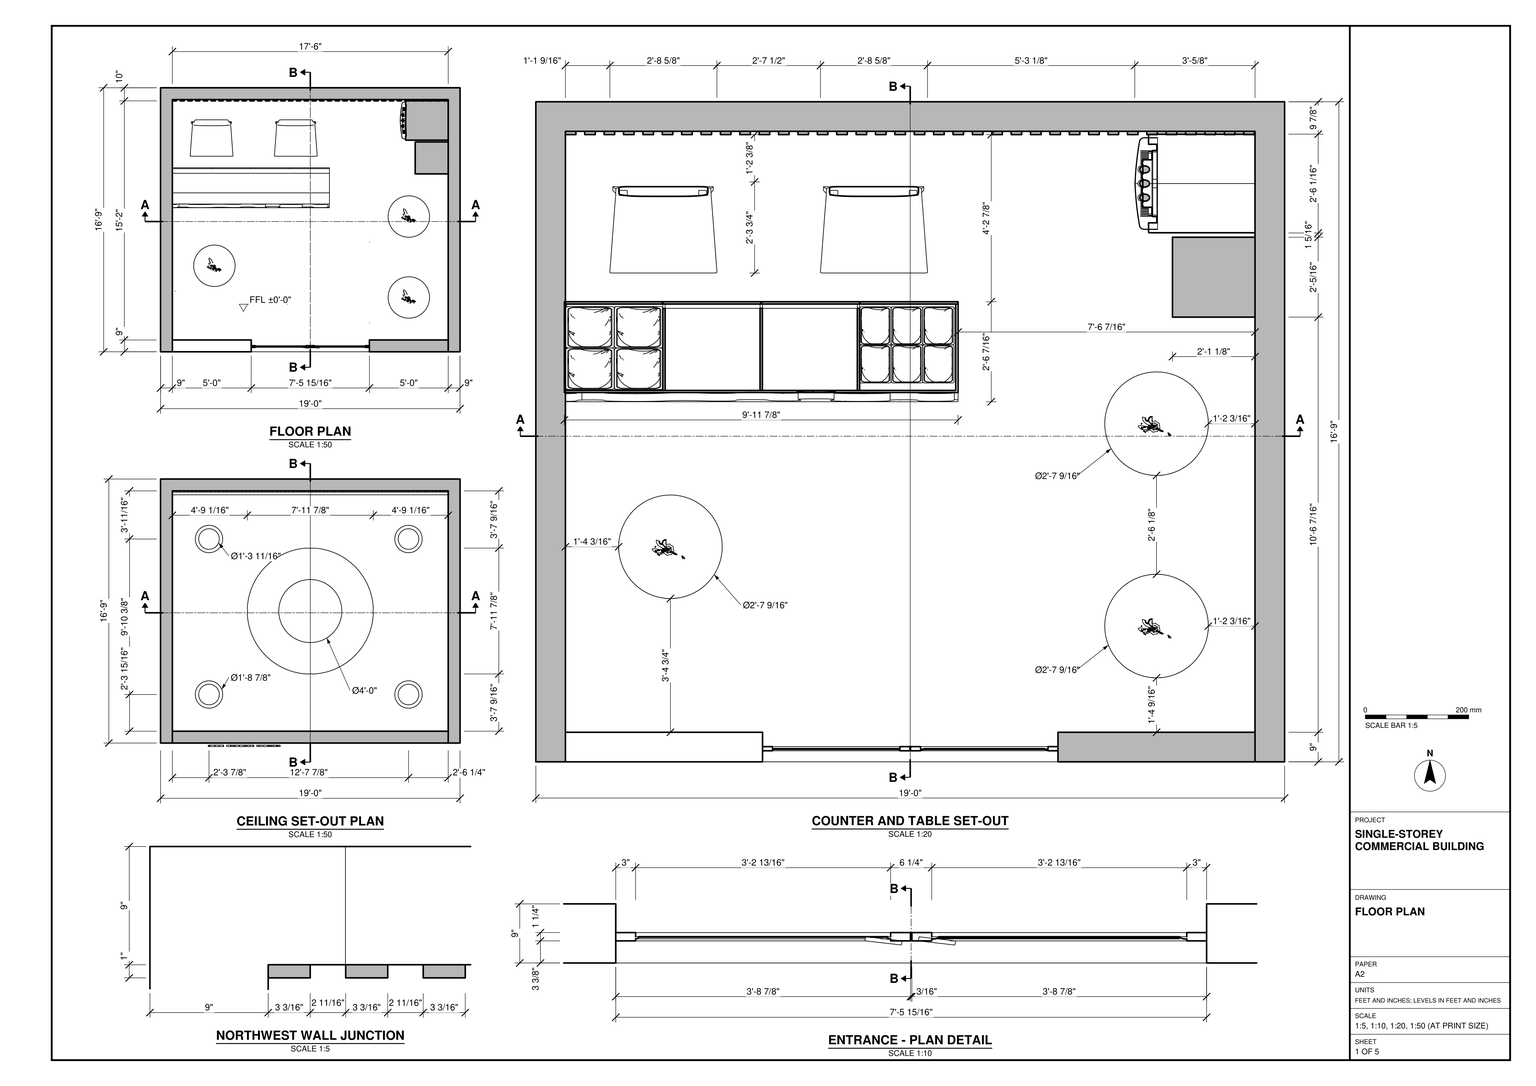
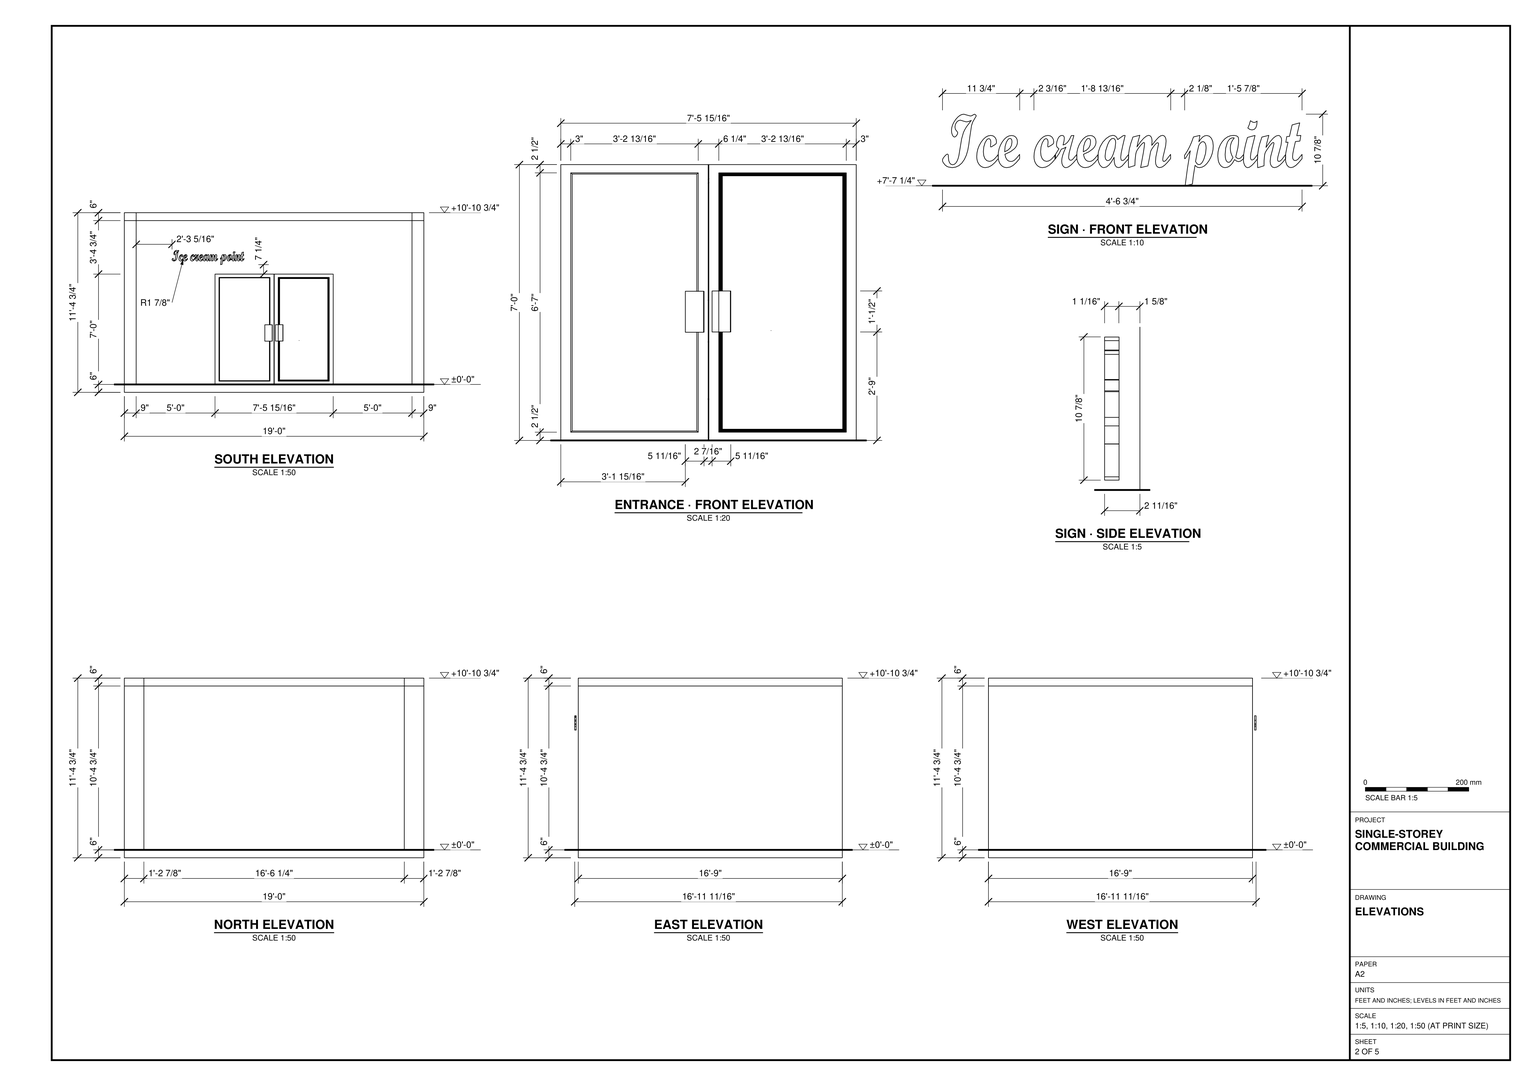
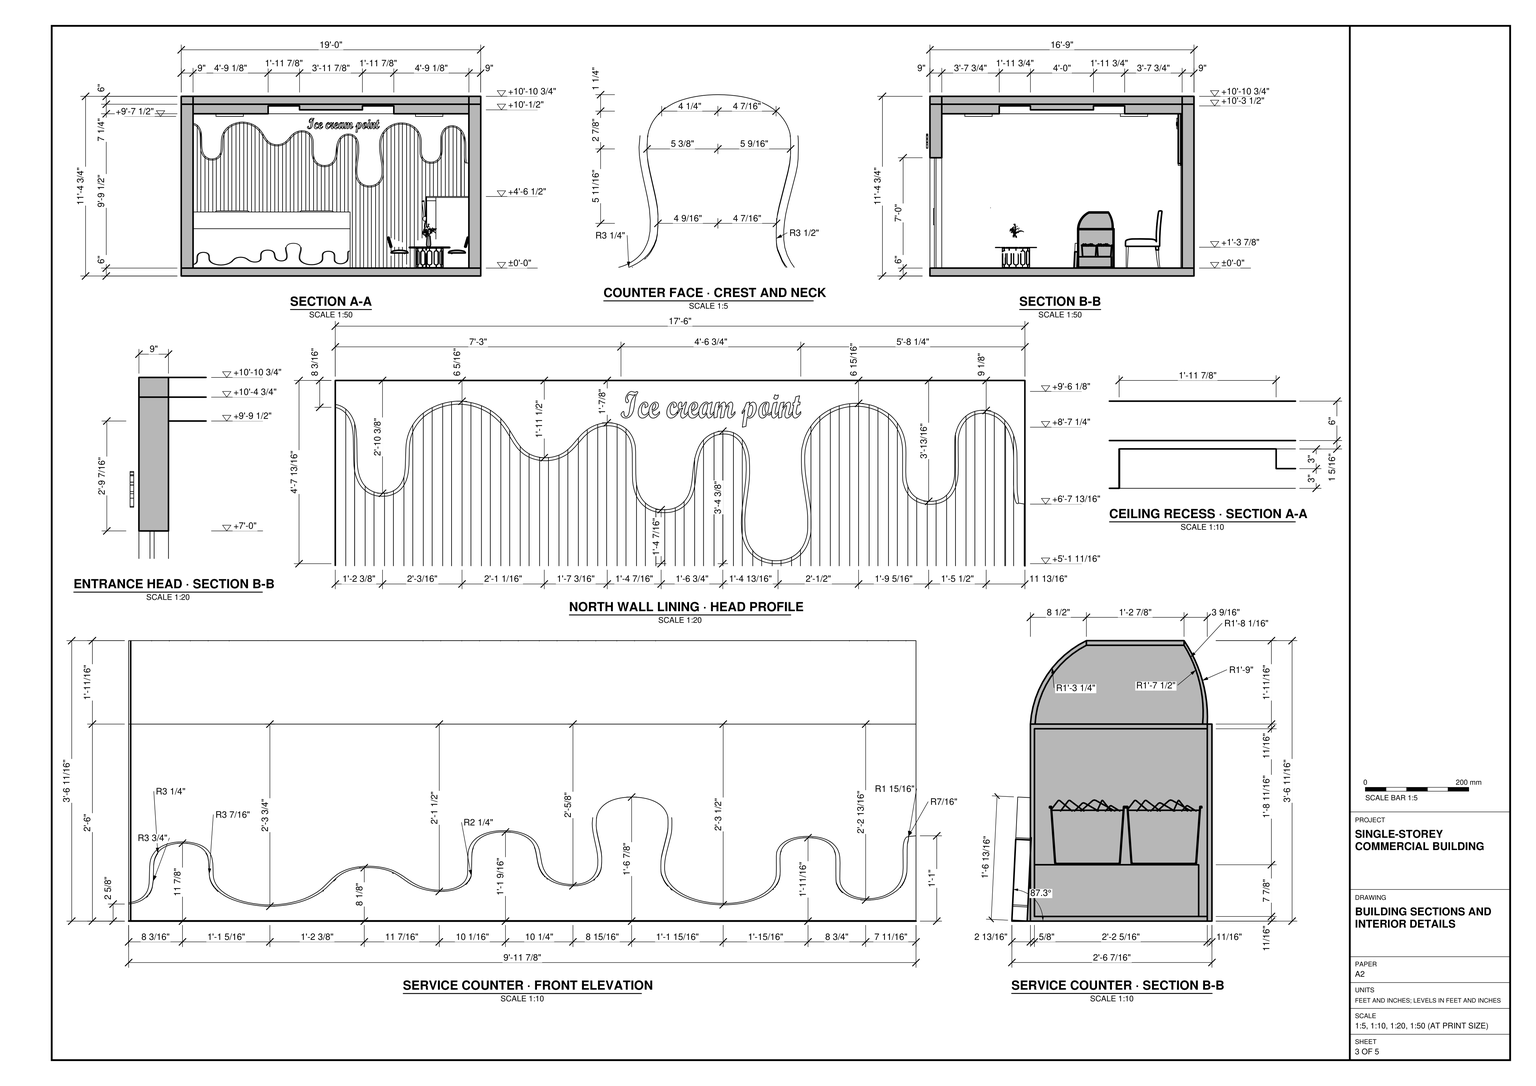
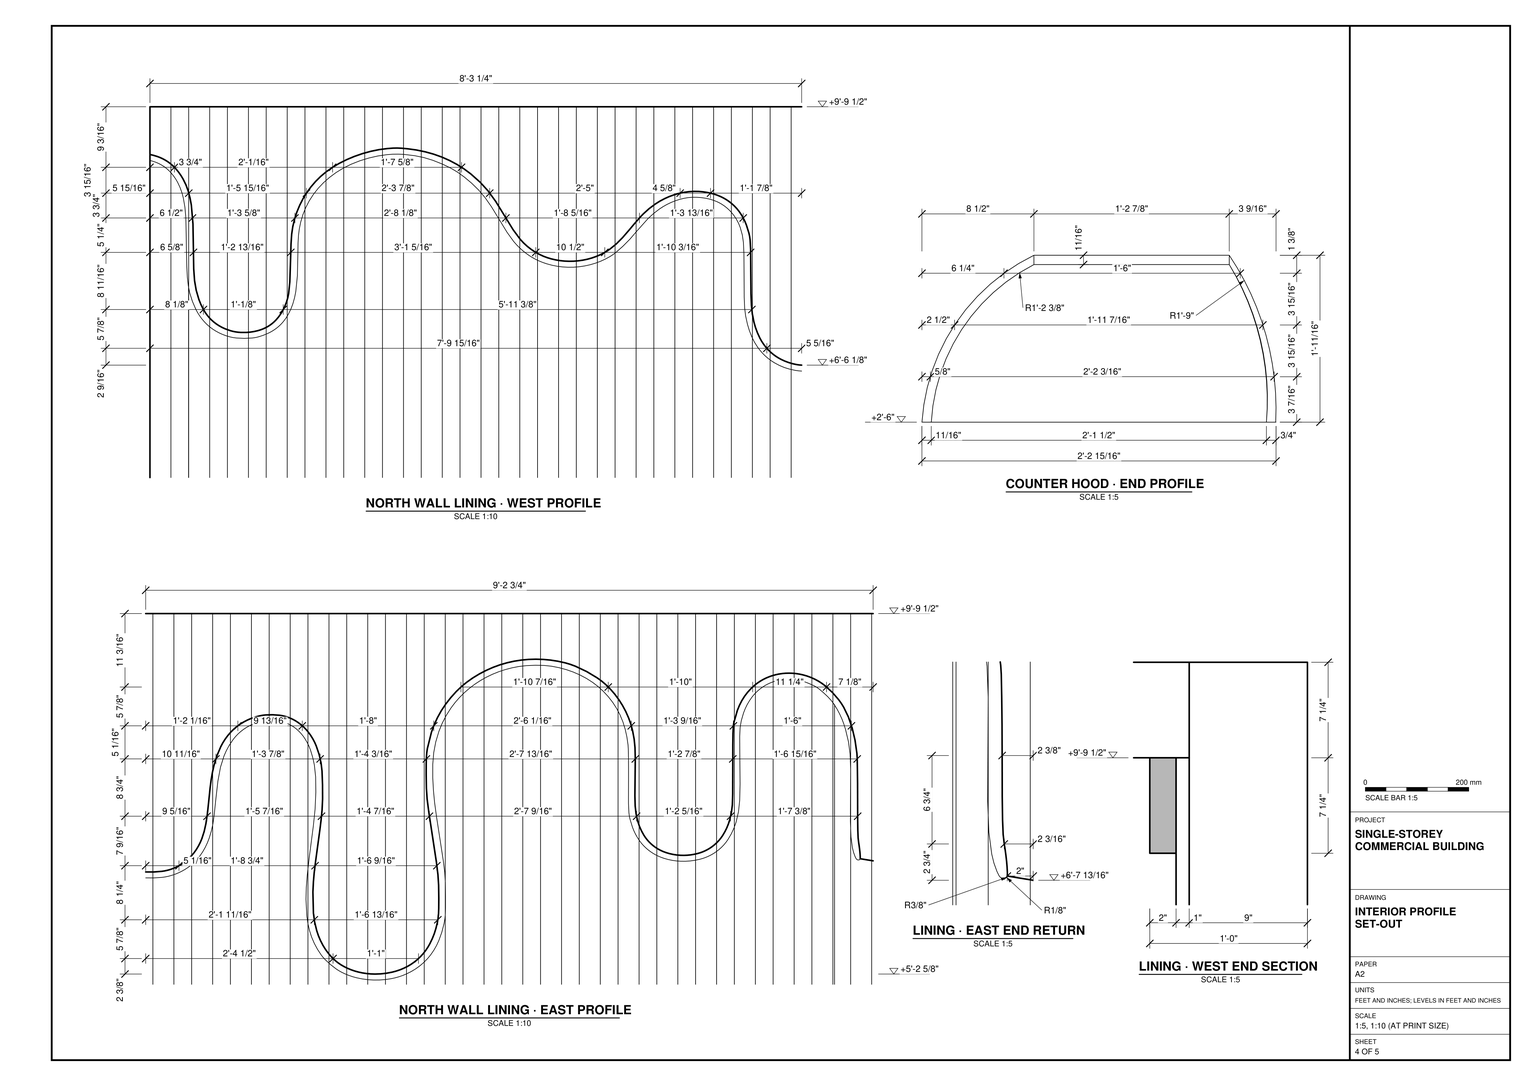
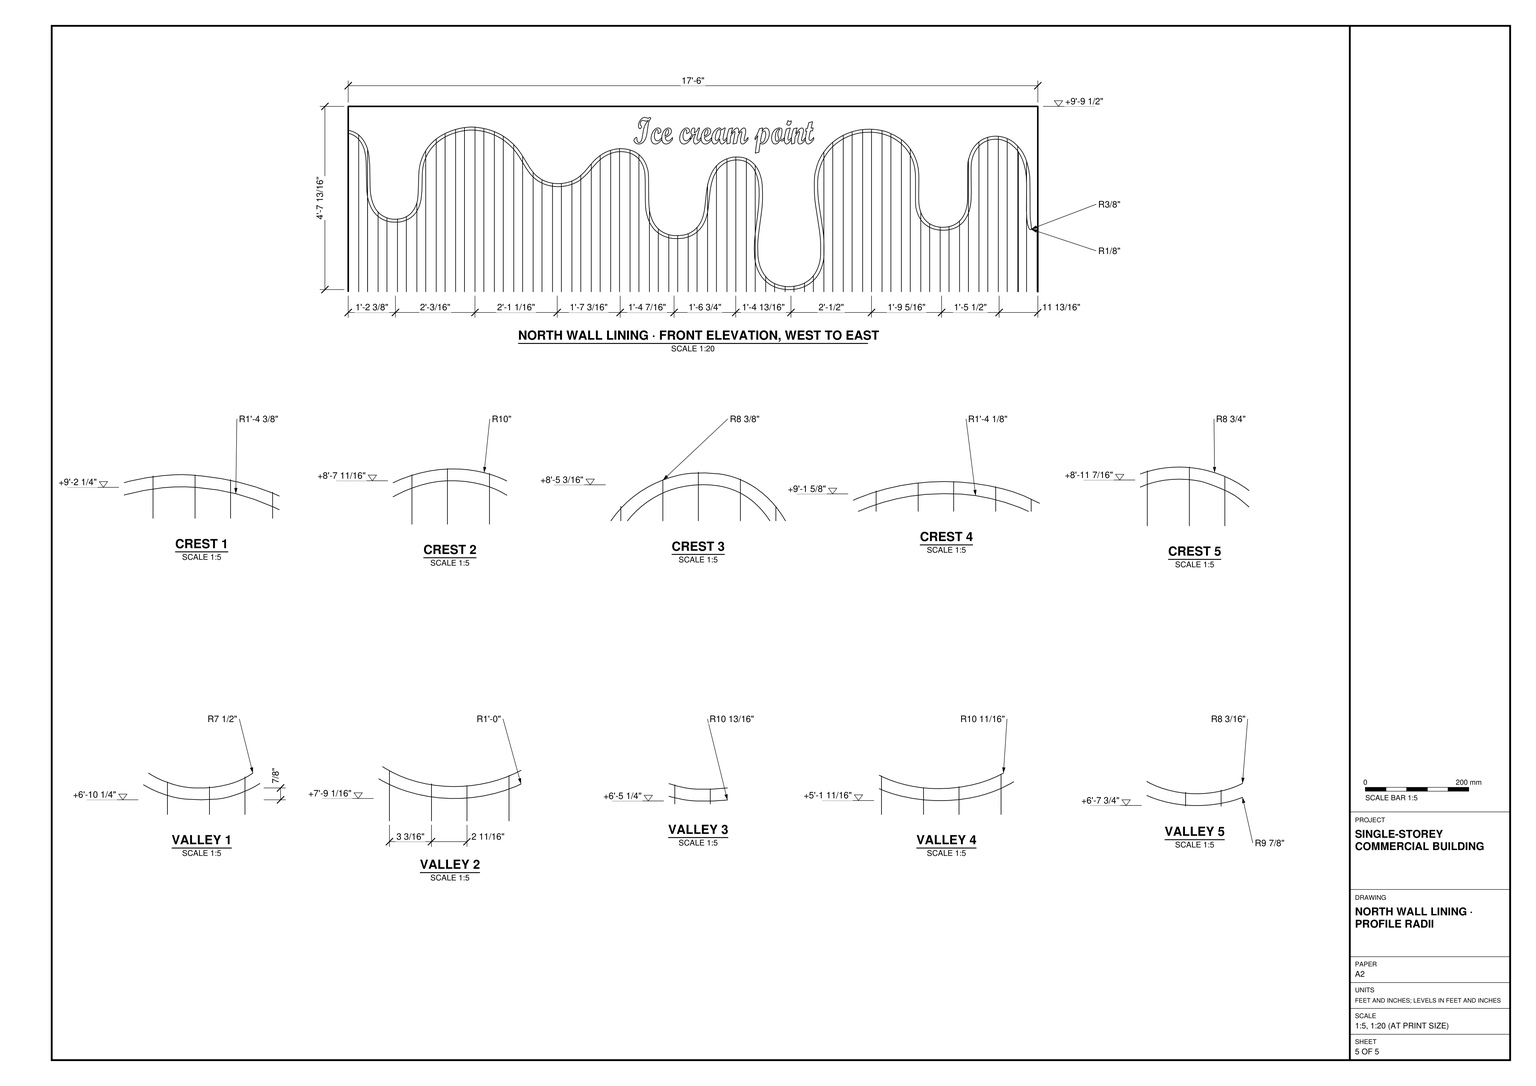
Build the ice cream shop in SketchUp from task_files/diagram_01.pdf. Work in feet and inches. The finished model, including the projecting entrance sign, must measure 19'-0" east to west, 16'-11 11/16" north to south and 11'-4 3/4" high. Set the single finished floor level at ±0'-0".

Build the floor slab, perimeter walls and flat roof slab. Use the wall thicknesses and north wall lining detail shown in plan. Centre the pair of framed entrance doors in the south wall, with pulls at the meeting edges. Place the exterior lettering above and to the left of the centre of the entrance as shown in elevation.

Use the counter and table set-out to arrange the interior. Run the display counter eastward from the west wall, leaving space for the two chairs between the counter and the north wall. Model the rounded display cover, the tubs and the undulating profile on the counter face. Behind it, form the full-width vertical wall lining with its varying curved head and interior lettering. Include the equipment and adjacent unit at the northeast corner. Place the three round tables in the customer area and reproduce the central and four surrounding circular features in the ceiling set-out.

Keep shell elements and each piece of furniture or joinery in separate groups or components, and use components for repeated parts. Decor and loose items may be any suitable library components. Save one SketchUp model as output_files/single_storey_ice_cream_shop_and_its_service_counter.skp.

# SketchUp Ruby script. Lengths in inches.
U = 1.inch
M = Sketchup.active_model
def pt(a) = Geom::Point3d.new(a.map { |v| v * U })
def face(e, loops, mat)
  f = e.add_face(loops[0].map { |a| pt(a) })
  loops[1..].each { |l| e.add_face(l.map { |a| pt(a) }).erase! }
  f.material = f.back_material = mat if mat
  f
end
# faces: each face lists its corners as indices into pts; further lists are holes
def faces(e, pts, list, mat = nil) = list.each { |f| face(e, (f[0].is_a?(Array) ? f : [f]).map { |l| l.map { |i| pts[i] } }, mat) }
# xy, xz, yz: faces in a plane at the given z, y or x. An outline is a flat list of corners, or four numbers for a rectangle; further outlines are holes
def ring(l) = l.size == 4 ? [[l[0], l[1]], [l[2], l[1]], [l[2], l[3]], [l[0], l[3]]] : l.each_slice(2).to_a
def flat(e, list, mat, &to3) = list.each { |f| face(e, (f[0].is_a?(Array) ? f : [f]).map { |l| ring(l).map { |u, v| to3.(u, v) } }, mat) }
def xy(e, z, list, mat = nil) = flat(e, list, mat) { |x, y| [x, y, z] }
def xz(e, y, list, mat = nil) = flat(e, list, mat) { |x, z| [x, y, z] }
def yz(e, x, list, mat = nil) = flat(e, list, mat) { |y, z| [x, y, z] }
def lines(e, pts, list) = list.each { |a, b| e.add_line(pt(pts[a]), pt(pts[b])) }
# prism: a flat outline (further loops are holes) pulled along v
def prism(e, loops, v, mat = nil)
  f = face(e, loops, mat); d = Geom::Vector3d.new(v.map { |x| x * U })
  f.pushpull(f.normal.samedirection?(d) ? d.length : -d.length)
end
def box(e, o, s, mat = nil) = prism(e, [[o, [o[0] + s[0], o[1], o[2]], [o[0] + s[0], o[1] + s[1], o[2]], [o[0], o[1] + s[1], o[2]]]], [0, 0, s[2]], mat)
def at(x, y, z, deg = 0) = Geom::Transformation.translation(pt([x, y, z])) * Geom::Transformation.rotation(ORIGIN, Z_AXIS, deg.degrees)
def axes(o, x, y, z) = Geom::Transformation.new([*x, 0, *y, 0, *z, 0, *pt(o).to_a, 1])
def part(name) = M.definitions.add(name)
# library, detail: a bought-in or finely detailed component or shape, given as its bounding box
def library(name, o, s) = part(name).tap { |d| box(d.entities, o, s) }
def detail(e, o, s) = box(e.add_group.entities, o, s)
def put(e, d, t, mat = nil) = e.add_instance(d, t).tap { |i| i.material = mat if mat }
def group(e, t, mat = nil) = e.add_group.tap { |g| g.transformation = t; g.material = mat if mat }.entities
root = M.entities
M.materials.add("Calacatta Gold (M2XN96)").color = [235, 228, 225]
M.materials.add("[Color A03]").color = [255, 101, 101]
M.materials.add("[Color C01]").color = [255, 229, 204]
M.materials.add("[Color_A02]").color = [255, 49, 49]
M.materials.add("미니냉장고").color = [225, 65, 65]
c1 = library("silla+generica",[-12.64,0.67,0],[23.23,30.27,48.95])
c2 = library("Untitled",[0,0,0],[82.62,78.29,61.04])
c3 = part("미니 냉장고\#1")
xy(c3.entities,0,[[1.57,0,7.48,14.96]],"[Color_A02]")
xy(c3.entities,25.59,[[0,0,9.06,14.96]])
xz(c3.entities,0,[[1.57,0,7.48,0,7.71,0.125,7.93,0.27,8.14,0.44,8.33,0.625,8.49,0.83,8.64,1.05,8.77,1.28,8.875,1.52,8.96,1.77,9.02,2.03,9.05,2.29,9.06,2.56,9.06,25.59,0,25.59,0,2.56,0.01,2.29,0.04,2.03,0.1,1.77,0.18,1.52,0.28,1.28,0.41,1.05,0.5625,0.83,0.73,0.625,0.92,0.44,1.12,0.27,1.34,0.125]],"[Color_A02]")
xz(c3.entities,14.96,[[1.57,0,1.34,0.125,1.12,0.27,0.92,0.44,0.73,0.625,0.5625,0.83,0.41,1.05,0.28,1.28,0.18,1.52,0.1,1.77,0.04,2.03,0.01,2.29,0,2.56,0,25.59,9.06,25.59,9.06,2.56,9.05,2.29,9.02,2.03,8.96,1.77,8.875,1.52,8.77,1.28,8.64,1.05,8.49,0.83,8.33,0.625,8.14,0.44,7.93,0.27,7.71,0.125,7.48,0]],"미니냉장고")
yz(c3.entities,0,[[0,2.56,14.96,25.59]],"미니냉장고")
yz(c3.entities,9.06,[[0,2.56,14.96,25.59]],"미니냉장고")
p = [[1.34,14.96,0.125],[1.57,14.96,0],[1.57,0,0],[1.34,0,0.125],[7.48,14.96,0],[7.71,14.96,0.125],
  [7.71,0,0.125],[7.48,0,0],[1.12,14.96,0.27],[1.12,0,0.27],[7.93,14.96,0.27],[7.93,0,0.27],
  [0.92,14.96,0.44],[0.92,0,0.44],[8.14,14.96,0.44],[8.14,0,0.44],[0.73,14.96,0.625],[0.73,0,0.625],
  [8.33,14.96,0.625],[8.33,0,0.625],[0.5625,14.96,0.83],[0.5625,0,0.83],[8.49,14.96,0.83],[8.49,0,0.83],
  [0.41,14.96,1.05],[0.41,0,1.05],[8.64,14.96,1.05],[8.64,0,1.05],[0.28,14.96,1.28],[0.28,0,1.28],
  [8.77,14.96,1.28],[8.77,0,1.28],[0.18,14.96,1.52],[0.18,0,1.52],[8.875,14.96,1.52],[8.875,0,1.52],
  [0.1,14.96,1.77],[0.1,0,1.77],[8.96,14.96,1.77],[8.96,0,1.77],[0.04,14.96,2.03],[0.04,0,2.03],
  [9.02,14.96,2.03],[9.02,0,2.03],[0.01,14.96,2.29],[0.01,0,2.29],[9.05,14.96,2.29],[9.05,0,2.29],
  [0,14.96,2.56],[0,0,2.56],[9.06,14.96,2.56],[9.06,0,2.56]]
faces(c3.entities,p,[[0,1,2,3],[4,5,6,7],[8,0,3,9],[5,10,11,6],[12,8,9,13],[10,14,15,11],[16,12,13,17],[14,18,19,15],
  [20,16,17,21],[18,22,23,19],[24,20,21,25],[22,26,27,23],[28,24,25,29],[26,30,31,27],[32,28,29,33],[30,34,35,31],
  [36,32,33,37],[34,38,39,35],[40,36,37,41],[38,42,43,39],[44,40,41,45],[42,46,47,43],[48,44,45,49],[46,50,51,47]],"[Color_A02]")
c4 = part("autocan")
put(c4.entities,c3,axes([0,14.96,25.59],[1,0,0],[0,-1,0],[0,0,-1]))
c5 = library("Untitled (1)",[52.61,1.75,0],[30.09,36.61,44.3125])
c6 = library("Group\#16",[0,0,0],[119.88,4.1,88.75])
c7 = library("Group\#25",[0,0,0],[119.88,30.46,42.71])
c8 = library("Group\#33",[0,0,0],[20.875,20.83,2])
c9 = library("Ice cream point",[0.1,0,0],[26.56,4.08,1])
c10 = library("Group\#2",[41.75,-69.27,0],[54.4,1.9,84])
put(root,c1,axes([40.28,148.24,-0.13],[1.4036,0,0],[0,0.9164,0],[0,0,0.8932]))
put(root,c1,axes([104.41,148.24,-0.13],[1.4036,0,0],[0,0.9164,0],[0,0,0.8932]))
put(root,c2,axes([9.01,36.14,0.11],[0.75,0,0],[0,0.75,0],[0,0,0.75]))
put(root,c2,axes([157.03,73.625,0.11],[0.75,0,0],[0,0.75,0],[0,0,0.75]))
put(root,c4,axes([193.86,159.76,0],[0,-2.688,0],[1.68,0,0],[0,0,2.1]))
put(root,c5,axes([180.63,243.76,0],[0,-1,0],[1,0,0],[0,0,1.23]))
put(root,c2,axes([157.03,12,0.11],[0.75,0,0],[0,0.75,0],[0,0,0.75]))
g1 = group(root,at(14.88,201,0),"[Color C01]")
xy(g1,0,[[-14.88,-201,-14.88,0,0,0,0,-9,-5.875,-9,-5.875,-201],[204.11,-201,204.11,-9,198.23,-9,198.23,0,213.12,0,213.12,-201],[0,-9,198.23,0]])
xy(g1,130.75,[[-14.88,-201,-5.875,-201,-5.875,-9,204.11,-9,204.11,-201,213.12,-201,213.12,0,-14.88,0]])
xz(g1,-201,[[-14.88,0,-5.875,130.75],[204.11,0,213.12,130.75]])
xz(g1,-9,[[-5.875,0,0,130.75],[0,0,198.23,130.75],[198.23,0,204.11,130.75]])
xz(g1,0,[[-14.88,0,0,130.75],[0,0,198.23,130.75],[198.23,0,213.12,130.75]])
yz(g1,-14.88,[[-201,0,0,130.75]])
yz(g1,-5.875,[[-201,0,-9,130.75]])
yz(g1,204.11,[[-201,0,-9,130.75]])
yz(g1,213.12,[[-201,0,0,130.75]])
put(root,c6,axes([9,187.9,0],[1.75172,0,0],[0,1,0],[0,0,1.32369]),"[Color C01]")
put(root,c7,at(8.7,109.65,0))
g2 = group(root,at(0,0,124.75),"[Color C01]")
xy(g2,0,[[0,0,228,201]])
xy(g2,6,[[0,0,228,201]],"[Color C01]")
xz(g2,0,[[0,0,228,6]])
xz(g2,201,[[0,0,228,6]])
yz(g2,0,[[0,0,201,6]])
yz(g2,228,[[0,0,201,6]])
g3 = group(root,at(9.01,0,124.75),"[Color C01]")
put(g3,c8,axes([17.43,144.91,-7.27],[1,0,0],[0,1,0],[0,0,-1]))
put(g3,c8,axes([169.31,26.54,-7.27],[1,0,0],[0,1,0],[0,0,-1]))
put(g3,c8,axes([169.31,144.91,-7.27],[1,0,0],[0,1,0],[0,0,-1]))
put(g3,c8,axes([17.43,26.54,-7.27],[1,0,0],[0,1,0],[0,0,-1]))
g4 = group(g3,at(0,0,-14))
xy(g4,6.73,[[[0,9,209.98,192],[102.48,52.57,99.97,52.76,97.48,53.09,95.01,53.55,92.57,54.14,90.16,54.85,87.79,55.6875,85.47,56.65,83.2,57.73,80.99,58.93,78.85,60.24,76.78,61.67,74.78,63.2,72.875,64.83,71.05,66.56,69.32,68.38,67.6875,70.29,66.16,72.29,64.74,74.36,63.42,76.5,62.22,78.71,61.14,80.98,60.18,83.3,59.34,85.67,58.63,88.08,58.04,90.52,57.58,92.99,57.26,95.48,57.06,97.99,57.26,100.5,57.06,103.01,57.26,105.52,57.58,108.01,58.04,110.48,58.63,112.92,59.34,115.33,60.18,117.7,61.14,120.02,62.22,122.29,63.42,124.5,64.74,126.64,66.16,128.71,67.6875,130.71,69.32,132.62,71.05,134.44,72.875,136.17,74.78,137.8,76.78,139.33,78.85,140.76,80.99,142.07,83.2,143.27,85.47,144.35,87.79,145.3125,90.16,146.15,92.57,146.86,95.01,147.45,97.48,147.91,99.97,148.24,102.48,148.43,104.99,148.24,107.5,148.43,110.01,148.24,112.5,147.91,114.97,147.45,117.42,146.86,119.83,146.15,122.19,145.3125,124.52,144.35,126.78,143.27,128.99,142.07,131.13,140.76,133.21,139.33,135.2,137.8,137.11,136.17,138.93,134.44,140.66,132.62,142.3,130.71,143.83,128.71,145.25,126.64,146.5625,124.5,147.76,122.29,148.84,120.02,149.8,117.7,150.64,115.33,151.36,112.92,151.94,110.48,152.4,108.01,152.73,105.52,152.93,103.01,152.73,100.5,152.93,97.99,152.73,95.48,152.4,92.99,151.94,90.52,151.36,88.08,150.64,85.67,149.8,83.3,148.84,80.98,147.76,78.71,146.5625,76.5,145.25,74.36,143.83,72.29,142.3,70.29,140.66,68.38,138.93,66.56,137.11,64.83,135.2,63.2,133.21,61.67,131.13,60.24,128.99,58.93,126.78,57.73,124.52,56.65,122.19,55.6875,119.83,54.85,117.42,54.14,114.97,53.55,112.5,53.09,110.01,52.76,107.5,52.57,104.99,52.76]]])
xy(g4,9.73,[[104.99,76.5,106.875,76.57,108.75,76.8,110.59,77.16,112.41,77.67,114.18,78.33,115.89,79.12,117.53,80.04,119.1,81.08,120.58,82.25,121.96,83.53,123.24,84.91,124.41,86.39,125.46,87.96,126.375,89.6,127.17,91.32,127.82,93.08,128.33,94.9,128.7,96.75,128.92,98.62,128.99,100.5,128.92,102.38,128.7,104.25,128.33,106.1,127.82,107.92,127.17,109.68,126.375,111.4,125.46,113.04,124.41,114.61,123.24,116.09,121.96,117.47,120.58,118.75,119.1,119.92,117.53,120.96,115.89,121.88,114.18,122.67,112.41,123.33,110.59,123.84,108.75,124.2,106.875,124.43,104.99,124.5,103.11,124.43,101.24,124.2,99.39,123.84,97.58,123.33,95.81,122.67,94.1,121.88,92.45,120.96,90.89,119.92,89.41,118.75,88.02,117.47,86.74,116.09,85.58,114.61,84.53,113.04,83.61,111.4,82.82,109.68,82.17,107.92,81.66,106.1,81.29,104.25,81.07,102.38,80.99,100.5,81.07,98.62,81.29,96.75,81.66,94.9,82.17,93.08,82.82,91.32,83.61,89.6,84.53,87.96,85.58,86.39,86.74,84.91,88.02,83.53,89.41,82.25,90.89,81.08,92.45,80.04,94.1,79.12,95.81,78.33,97.58,77.67,99.39,77.16,101.24,76.8,103.11,76.57]])
xy(g4,12.73,[[[102.48,52.57,104.99,52.76,107.5,52.57,110.01,52.76,112.5,53.09,114.97,53.55,117.42,54.14,119.83,54.85,122.19,55.6875,124.52,56.65,126.78,57.73,128.99,58.93,131.13,60.24,133.21,61.67,135.2,63.2,137.11,64.83,138.93,66.56,140.66,68.38,142.3,70.29,143.83,72.29,145.25,74.36,146.5625,76.5,147.76,78.71,148.84,80.98,149.8,83.3,150.64,85.67,151.36,88.08,151.94,90.52,152.4,92.99,152.73,95.48,152.93,97.99,152.73,100.5,152.93,103.01,152.73,105.52,152.4,108.01,151.94,110.48,151.36,112.92,150.64,115.33,149.8,117.7,148.84,120.02,147.76,122.29,146.5625,124.5,145.25,126.64,143.83,128.71,142.3,130.71,140.66,132.62,138.93,134.44,137.11,136.17,135.2,137.8,133.21,139.33,131.13,140.76,128.99,142.07,126.78,143.27,124.52,144.35,122.19,145.3125,119.83,146.15,117.42,146.86,114.97,147.45,112.5,147.91,110.01,148.24,107.5,148.43,104.99,148.24,102.48,148.43,99.97,148.24,97.48,147.91,95.01,147.45,92.57,146.86,90.16,146.15,87.79,145.3125,85.47,144.35,83.2,143.27,80.99,142.07,78.85,140.76,76.78,139.33,74.78,137.8,72.875,136.17,71.05,134.44,69.32,132.62,67.6875,130.71,66.16,128.71,64.74,126.64,63.42,124.5,62.22,122.29,61.14,120.02,60.18,117.7,59.34,115.33,58.63,112.92,58.04,110.48,57.58,108.01,57.26,105.52,57.06,103.01,57.26,100.5,57.06,97.99,57.26,95.48,57.58,92.99,58.04,90.52,58.63,88.08,59.34,85.67,60.18,83.3,61.14,80.98,62.22,78.71,63.42,76.5,64.74,74.36,66.16,72.29,67.6875,70.29,69.32,68.38,71.05,66.56,72.875,64.83,74.78,63.2,76.78,61.67,78.85,60.24,80.99,58.93,83.2,57.73,85.47,56.65,87.79,55.6875,90.16,54.85,92.57,54.14,95.01,53.55,97.48,53.09,99.97,52.76],[104.99,76.5,103.11,76.57,101.24,76.8,99.39,77.16,97.58,77.67,95.81,78.33,94.1,79.12,92.45,80.04,90.89,81.08,89.41,82.25,88.02,83.53,86.74,84.91,85.58,86.39,84.53,87.96,83.61,89.6,82.82,91.32,82.17,93.08,81.66,94.9,81.29,96.75,81.07,98.62,80.99,100.5,81.07,102.38,81.29,104.25,81.66,106.1,82.17,107.92,82.82,109.68,83.61,111.4,84.53,113.04,85.58,114.61,86.74,116.09,88.02,117.47,89.41,118.75,90.89,119.92,92.45,120.96,94.1,121.88,95.81,122.67,97.58,123.33,99.39,123.84,101.24,124.2,103.11,124.43,104.99,124.5,106.875,124.43,108.75,124.2,110.59,123.84,112.41,123.33,114.18,122.67,115.89,121.88,117.53,120.96,119.1,119.92,120.58,118.75,121.96,117.47,123.24,116.09,124.41,114.61,125.46,113.04,126.375,111.4,127.17,109.68,127.82,107.92,128.33,106.1,128.7,104.25,128.92,102.38,128.99,100.5,128.92,98.62,128.7,96.75,128.33,94.9,127.82,93.08,127.17,91.32,126.375,89.6,125.46,87.96,124.41,86.39,123.24,84.91,121.96,83.53,120.58,82.25,119.1,81.08,117.53,80.04,115.89,79.12,114.18,78.33,112.41,77.67,110.59,77.16,108.75,76.8,106.875,76.57]]])
xy(g4,14,[[0,9,209.98,192]])
xz(g4,9,[[0,6.73,209.98,14]])
xz(g4,192,[[0,6.73,209.98,14]])
yz(g4,0,[[9,6.73,192,14]])
yz(g4,209.98,[[9,6.73,192,14]])
p = [[99.97,52.76,6.73],[102.48,52.57,6.73],[102.48,52.57,12.73],[99.97,52.76,12.73],[104.99,52.76,6.73],[104.99,52.76,12.73],
  [107.5,52.57,6.73],[107.5,52.57,12.73],[110.01,52.76,6.73],[110.01,52.76,12.73],[97.48,53.09,6.73],[97.48,53.09,12.73],
  [112.5,53.09,6.73],[112.5,53.09,12.73],[95.01,53.55,6.73],[95.01,53.55,12.73],[114.97,53.55,6.73],[114.97,53.55,12.73],
  [92.57,54.14,6.73],[92.57,54.14,12.73],[117.42,54.14,6.73],[117.42,54.14,12.73],[90.16,54.85,6.73],[90.16,54.85,12.73],
  [119.83,54.85,6.73],[119.83,54.85,12.73],[87.79,55.6875,6.73],[87.79,55.6875,12.73],[122.19,55.6875,6.73],[122.19,55.6875,12.73],
  [85.47,56.65,6.73],[85.47,56.65,12.73],[124.52,56.65,6.73],[124.52,56.65,12.73],[83.2,57.73,6.73],[83.2,57.73,12.73],
  [126.78,57.73,6.73],[126.78,57.73,12.73],[80.99,58.93,6.73],[80.99,58.93,12.73],[128.99,58.93,6.73],[128.99,58.93,12.73],
  [78.85,60.24,6.73],[78.85,60.24,12.73],[131.13,60.24,6.73],[131.13,60.24,12.73],[76.78,61.67,6.73],[76.78,61.67,12.73],
  [133.21,61.67,6.73],[133.21,61.67,12.73],[74.78,63.2,6.73],[74.78,63.2,12.73],[135.2,63.2,6.73],[135.2,63.2,12.73],
  [72.875,64.83,6.73],[72.875,64.83,12.73],[137.11,64.83,6.73],[137.11,64.83,12.73],[71.05,66.56,6.73],[71.05,66.56,12.73],
  [138.93,66.56,6.73],[138.93,66.56,12.73],[69.32,68.38,6.73],[69.32,68.38,12.73],[140.66,68.38,6.73],[140.66,68.38,12.73],
  [67.6875,70.29,6.73],[67.6875,70.29,12.73],[142.3,70.29,6.73],[142.3,70.29,12.73],[66.16,72.29,6.73],[66.16,72.29,12.73],
  [143.83,72.29,6.73],[143.83,72.29,12.73],[64.74,74.36,6.73],[64.74,74.36,12.73],[145.25,74.36,6.73],[145.25,74.36,12.73],
  [63.42,76.5,6.73],[63.42,76.5,12.73],[146.5625,76.5,6.73],[146.5625,76.5,12.73],[62.22,78.71,6.73],[62.22,78.71,12.73],
  [147.76,78.71,6.73],[147.76,78.71,12.73],[61.14,80.98,6.73],[61.14,80.98,12.73],[148.84,80.98,6.73],[148.84,80.98,12.73],
  [60.18,83.3,6.73],[60.18,83.3,12.73],[149.8,83.3,6.73],[149.8,83.3,12.73],[59.34,85.67,6.73],[59.34,85.67,12.73],
  [150.64,85.67,6.73],[150.64,85.67,12.73],[58.63,88.08,6.73],[58.63,88.08,12.73],[151.36,88.08,6.73],[151.36,88.08,12.73],
  [58.04,90.52,6.73],[58.04,90.52,12.73],[151.94,90.52,6.73],[151.94,90.52,12.73],[57.58,92.99,6.73],[57.58,92.99,12.73],
  [152.4,92.99,6.73],[152.4,92.99,12.73],[57.26,95.48,6.73],[57.26,95.48,12.73],[152.73,95.48,6.73],[152.73,95.48,12.73],
  [57.06,97.99,6.73],[57.06,97.99,12.73],[152.93,97.99,6.73],[152.93,97.99,12.73],[57.26,100.5,6.73],[57.26,100.5,12.73],
  [152.73,100.5,6.73],[152.73,100.5,12.73],[57.06,103.01,6.73],[57.06,103.01,12.73],[152.93,103.01,6.73],[152.93,103.01,12.73],
  [57.26,105.52,6.73],[57.26,105.52,12.73],[152.73,105.52,6.73],[152.73,105.52,12.73],[57.58,108.01,6.73],[57.58,108.01,12.73],
  [152.4,108.01,6.73],[152.4,108.01,12.73],[58.04,110.48,6.73],[58.04,110.48,12.73],[151.94,110.48,6.73],[151.94,110.48,12.73],
  [58.63,112.92,6.73],[58.63,112.92,12.73],[151.36,112.92,6.73],[151.36,112.92,12.73],[59.34,115.33,6.73],[59.34,115.33,12.73],
  [150.64,115.33,6.73],[150.64,115.33,12.73],[60.18,117.7,6.73],[60.18,117.7,12.73],[149.8,117.7,6.73],[149.8,117.7,12.73],
  [61.14,120.02,6.73],[61.14,120.02,12.73],[148.84,120.02,6.73],[148.84,120.02,12.73],[62.22,122.29,6.73],[62.22,122.29,12.73],
  [147.76,122.29,6.73],[147.76,122.29,12.73],[63.42,124.5,6.73],[63.42,124.5,12.73],[146.5625,124.5,6.73],[146.5625,124.5,12.73],
  [64.74,126.64,6.73],[64.74,126.64,12.73],[145.25,126.64,6.73],[145.25,126.64,12.73],[66.16,128.71,6.73],[66.16,128.71,12.73],
  [143.83,128.71,6.73],[143.83,128.71,12.73],[67.6875,130.71,6.73],[67.6875,130.71,12.73],[142.3,130.71,6.73],[142.3,130.71,12.73],
  [69.32,132.62,6.73],[69.32,132.62,12.73],[140.66,132.62,6.73],[140.66,132.62,12.73],[71.05,134.44,6.73],[71.05,134.44,12.73],
  [138.93,134.44,6.73],[138.93,134.44,12.73],[72.875,136.17,6.73],[72.875,136.17,12.73],[137.11,136.17,6.73],[137.11,136.17,12.73],
  [74.78,137.8,6.73],[74.78,137.8,12.73],[135.2,137.8,6.73],[135.2,137.8,12.73],[76.78,139.33,6.73],[76.78,139.33,12.73],
  [133.21,139.33,6.73],[133.21,139.33,12.73],[78.85,140.76,6.73],[78.85,140.76,12.73],[131.13,140.76,6.73],[131.13,140.76,12.73],
  [80.99,142.07,6.73],[80.99,142.07,12.73],[128.99,142.07,6.73],[128.99,142.07,12.73],[83.2,143.27,6.73],[83.2,143.27,12.73],
  [126.78,143.27,6.73],[126.78,143.27,12.73],[85.47,144.35,6.73],[85.47,144.35,12.73],[124.52,144.35,6.73],[124.52,144.35,12.73],
  [87.79,145.3125,6.73],[87.79,145.3125,12.73],[122.19,145.3125,6.73],[122.19,145.3125,12.73],[90.16,146.15,6.73],[90.16,146.15,12.73],
  [119.83,146.15,6.73],[119.83,146.15,12.73],[92.57,146.86,6.73],[92.57,146.86,12.73],[117.42,146.86,6.73],[117.42,146.86,12.73],
  [95.01,147.45,6.73],[95.01,147.45,12.73],[114.97,147.45,6.73],[114.97,147.45,12.73],[97.48,147.91,6.73],[97.48,147.91,12.73],
  [112.5,147.91,6.73],[112.5,147.91,12.73],[99.97,148.24,6.73],[99.97,148.24,12.73],[110.01,148.24,6.73],[110.01,148.24,12.73],
  [102.48,148.43,6.73],[102.48,148.43,12.73],[104.99,148.24,6.73],[104.99,148.24,12.73],[107.5,148.43,6.73],[107.5,148.43,12.73],
  [104.99,76.5,9.73],[103.11,76.57,9.73],[103.11,76.57,12.73],[104.99,76.5,12.73],[106.875,76.57,9.73],[106.875,76.57,12.73],
  [101.24,76.8,9.73],[101.24,76.8,12.73],[108.75,76.8,9.73],[108.75,76.8,12.73],[99.39,77.16,9.73],[99.39,77.16,12.73],
  [110.59,77.16,9.73],[110.59,77.16,12.73],[97.58,77.67,9.73],[97.58,77.67,12.73],[112.41,77.67,9.73],[112.41,77.67,12.73],
  [95.81,78.33,9.73],[95.81,78.33,12.73],[114.18,78.33,9.73],[114.18,78.33,12.73],[94.1,79.12,9.73],[94.1,79.12,12.73],
  [115.89,79.12,9.73],[115.89,79.12,12.73],[92.45,80.04,9.73],[92.45,80.04,12.73],[117.53,80.04,9.73],[117.53,80.04,12.73],
  [90.89,81.08,9.73],[90.89,81.08,12.73],[119.1,81.08,9.73],[119.1,81.08,12.73],[89.41,82.25,9.73],[89.41,82.25,12.73],
  [120.58,82.25,9.73],[120.58,82.25,12.73],[88.02,83.53,9.73],[88.02,83.53,12.73],[121.96,83.53,9.73],[121.96,83.53,12.73],
  [86.74,84.91,9.73],[86.74,84.91,12.73],[123.24,84.91,9.73],[123.24,84.91,12.73],[85.58,86.39,9.73],[85.58,86.39,12.73],
  [124.41,86.39,9.73],[124.41,86.39,12.73],[84.53,87.96,9.73],[84.53,87.96,12.73],[125.46,87.96,9.73],[125.46,87.96,12.73],
  [83.61,89.6,9.73],[83.61,89.6,12.73],[126.375,89.6,9.73],[126.375,89.6,12.73],[82.82,91.32,9.73],[82.82,91.32,12.73],
  [127.17,91.32,9.73],[127.17,91.32,12.73],[82.17,93.08,9.73],[82.17,93.08,12.73],[127.82,93.08,9.73],[127.82,93.08,12.73],
  [81.66,94.9,9.73],[81.66,94.9,12.73],[128.33,94.9,9.73],[128.33,94.9,12.73],[81.29,96.75,9.73],[81.29,96.75,12.73],
  [128.7,96.75,9.73],[128.7,96.75,12.73],[81.07,98.62,9.73],[81.07,98.62,12.73],[128.92,98.62,9.73],[128.92,98.62,12.73],
  [80.99,100.5,9.73],[80.99,100.5,12.73],[128.99,100.5,9.73],[128.99,100.5,12.73],[81.07,102.38,9.73],[81.07,102.38,12.73],
  [128.92,102.38,9.73],[128.92,102.38,12.73],[81.29,104.25,9.73],[81.29,104.25,12.73],[128.7,104.25,9.73],[128.7,104.25,12.73],
  [81.66,106.1,9.73],[81.66,106.1,12.73],[128.33,106.1,9.73],[128.33,106.1,12.73],[82.17,107.92,9.73],[82.17,107.92,12.73],
  [127.82,107.92,9.73],[127.82,107.92,12.73],[82.82,109.68,9.73],[82.82,109.68,12.73],[127.17,109.68,9.73],[127.17,109.68,12.73],
  [83.61,111.4,9.73],[83.61,111.4,12.73],[126.375,111.4,9.73],[126.375,111.4,12.73],[84.53,113.04,9.73],[84.53,113.04,12.73],
  [125.46,113.04,9.73],[125.46,113.04,12.73],[85.58,114.61,9.73],[85.58,114.61,12.73],[124.41,114.61,9.73],[124.41,114.61,12.73],
  [86.74,116.09,9.73],[86.74,116.09,12.73],[123.24,116.09,9.73],[123.24,116.09,12.73],[88.02,117.47,9.73],[88.02,117.47,12.73],
  [121.96,117.47,9.73],[121.96,117.47,12.73],[89.41,118.75,9.73],[89.41,118.75,12.73],[120.58,118.75,9.73],[120.58,118.75,12.73],
  [90.89,119.92,9.73],[90.89,119.92,12.73],[119.1,119.92,9.73],[119.1,119.92,12.73],[92.45,120.96,9.73],[92.45,120.96,12.73],
  [117.53,120.96,9.73],[117.53,120.96,12.73],[94.1,121.88,9.73],[94.1,121.88,12.73],[115.89,121.88,9.73],[115.89,121.88,12.73],
  [95.81,122.67,9.73],[95.81,122.67,12.73],[114.18,122.67,9.73],[114.18,122.67,12.73],[97.58,123.33,9.73],[97.58,123.33,12.73],
  [112.41,123.33,9.73],[112.41,123.33,12.73],[99.39,123.84,9.73],[99.39,123.84,12.73],[110.59,123.84,9.73],[110.59,123.84,12.73],
  [101.24,124.2,9.73],[101.24,124.2,12.73],[108.75,124.2,9.73],[108.75,124.2,12.73],[103.11,124.43,9.73],[103.11,124.43,12.73],
  [106.875,124.43,9.73],[106.875,124.43,12.73],[104.99,124.5,9.73],[104.99,124.5,12.73],[209.98,0,0],[209.98,9,0],
  [0,9,0],[0,0,0]]
faces(g4,p,[[0,1,2,3],[1,4,5,2],[4,6,7,5],[6,8,9,7],[10,0,3,11],[8,12,13,9],[14,10,11,15],[12,16,17,13],
  [18,14,15,19],[16,20,21,17],[22,18,19,23],[20,24,25,21],[26,22,23,27],[24,28,29,25],[30,26,27,31],[28,32,33,29],
  [34,30,31,35],[32,36,37,33],[38,34,35,39],[36,40,41,37],[42,38,39,43],[40,44,45,41],[46,42,43,47],[44,48,49,45],
  [50,46,47,51],[48,52,53,49],[54,50,51,55],[52,56,57,53],[58,54,55,59],[56,60,61,57],[62,58,59,63],[60,64,65,61],
  [66,62,63,67],[64,68,69,65],[70,66,67,71],[68,72,73,69],[74,70,71,75],[72,76,77,73],[78,74,75,79],[76,80,81,77],
  [82,78,79,83],[80,84,85,81],[86,82,83,87],[84,88,89,85],[90,86,87,91],[88,92,93,89],[94,90,91,95],[92,96,97,93],
  [98,94,95,99],[96,100,101,97],[102,98,99,103],[100,104,105,101],[106,102,103,107],[104,108,109,105],[110,106,107,111],[108,112,113,109],
  [114,110,111,115],[112,116,117,113],[118,114,115,119],[116,120,121,117],[122,118,119,123],[120,124,125,121],[126,122,123,127],[124,128,129,125],
  [130,126,127,131],[128,132,133,129],[134,130,131,135],[132,136,137,133],[138,134,135,139],[136,140,141,137],[142,138,139,143],[140,144,145,141],
  [146,142,143,147],[144,148,149,145],[150,146,147,151],[148,152,153,149],[154,150,151,155],[152,156,157,153],[158,154,155,159],[156,160,161,157],
  [162,158,159,163],[160,164,165,161],[166,162,163,167],[164,168,169,165],[170,166,167,171],[168,172,173,169],[174,170,171,175],[172,176,177,173],
  [178,174,175,179],[176,180,181,177],[182,178,179,183],[180,184,185,181],[186,182,183,187],[184,188,189,185],[190,186,187,191],[188,192,193,189],
  [194,190,191,195],[192,196,197,193],[198,194,195,199],[196,200,201,197],[202,198,199,203],[200,204,205,201],[206,202,203,207],[204,208,209,205],
  [210,206,207,211],[208,212,213,209],[214,210,211,215],[212,216,217,213],[218,214,215,219],[216,220,221,217],[222,218,219,223],[220,224,225,221],
  [226,222,223,227],[224,228,229,225],[230,226,227,231],[228,232,233,229],[234,230,231,235],[236,234,235,237],[238,236,237,239],[232,238,239,233],
  [240,241,242,243],[244,240,243,245],[241,246,247,242],[248,244,245,249],[246,250,251,247],[252,248,249,253],[250,254,255,251],[256,252,253,257],
  [254,258,259,255],[260,256,257,261],[258,262,263,259],[264,260,261,265],[262,266,267,263],[268,264,265,269],[266,270,271,267],[272,268,269,273],
  [270,274,275,271],[276,272,273,277],[274,278,279,275],[280,276,277,281],[278,282,283,279],[284,280,281,285],[282,286,287,283],[288,284,285,289],
  [286,290,291,287],[292,288,289,293],[290,294,295,291],[296,292,293,297],[294,298,299,295],[300,296,297,301],[298,302,303,299],[304,300,301,305],
  [302,306,307,303],[308,304,305,309],[306,310,311,307],[312,308,309,313],[310,314,315,311],[316,312,313,317],[314,318,319,315],[320,316,317,321],
  [318,322,323,319],[324,320,321,325],[322,326,327,323],[328,324,325,329],[326,330,331,327],[332,328,329,333],[330,334,335,331],[336,332,333,337],
  [334,338,339,335],[340,336,337,341],[338,342,343,339],[344,340,341,345],[342,346,347,343],[348,344,345,349],[346,350,351,347],[352,348,349,353],
  [350,354,355,351],[356,352,353,357],[354,358,359,355],[360,356,357,361],[358,362,363,359],[364,360,361,365],[362,366,367,363],[368,364,365,369],
  [366,370,371,367],[372,368,369,373],[370,374,375,371],[376,372,373,377],[374,378,379,375],[380,376,377,381],[378,382,383,379],[384,380,381,385],
  [382,386,387,383],[388,384,385,389],[386,390,391,387],[392,388,389,393],[390,394,395,391],[396,392,393,397],[394,398,399,395],[398,396,397,399]])
lines(g4,p,[[400,401],[402,403]])
g5 = group(root,at(0,0,0),"[Color C01]")
box(g5,[0,0,-6],[228,201,6])
g6 = group(root,at(9.01,0,0))
put(g6,c9,axes([27.1,-1.59,91.22],[2.06177,0,0],[0,0,2.66882],[0,-1.1,0]),"[Color A03]")
put(g6,c10,axes([-9.01,72,0],[1.65364,0,0],[0,1,0],[0,0,1]),"Calacatta Gold (M2XN96)")
g7 = group(g6,at(0,9,0),"[Color C01]")
prism(g7,[[[209.98,0,0],[149.98,0,0],[149.98,0,84],[60.03,0,84],[60.03,0,0],[0,0,0],[0,0,130.75],[209.98,0,130.75]]],[0,-9,0],"[Color C01]")
